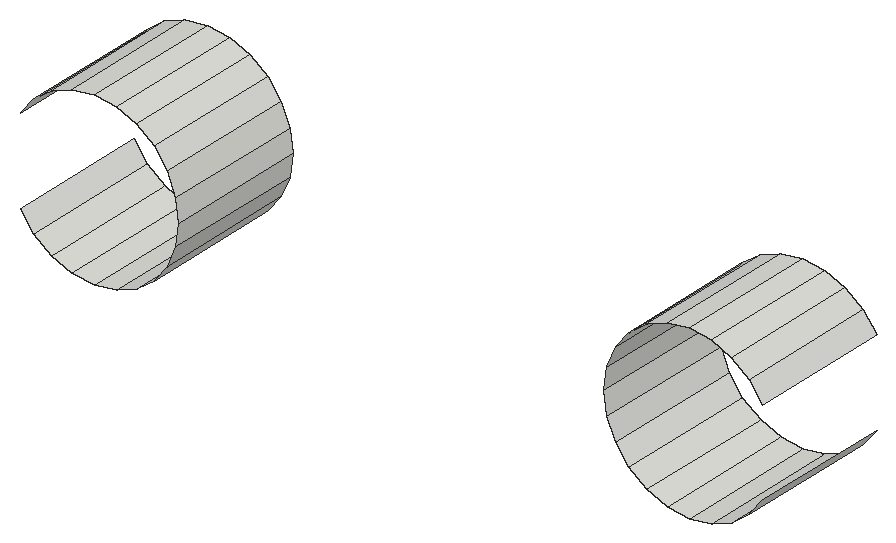
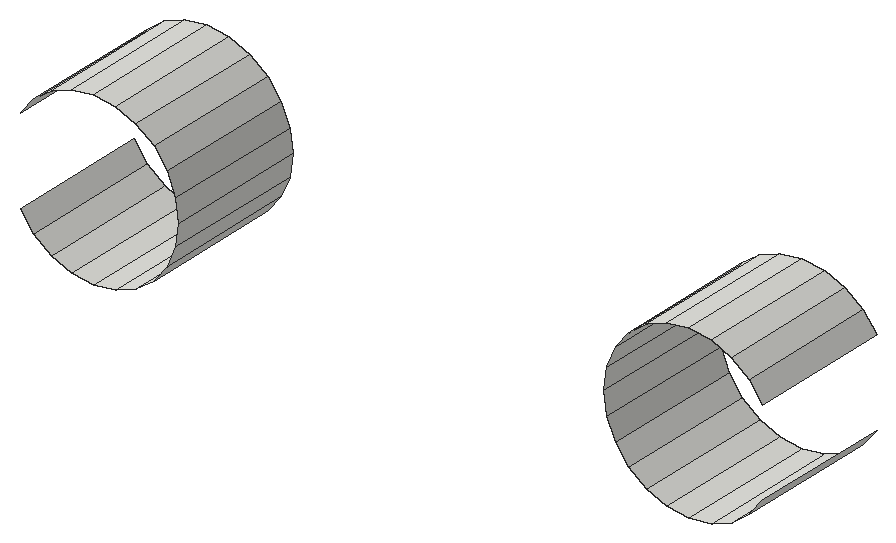
# SketchUp Ruby script. Lengths in inches.
U = 1.inch
M = Sketchup.active_model
def pt(a) = Geom::Point3d.new(a.map { |v| v * U })
def face(e, loops, mat)
  f = e.add_face(loops[0].map { |a| pt(a) })
  loops[1..].each { |l| e.add_face(l.map { |a| pt(a) }).erase! }
  f.material = f.back_material = mat if mat
  f
end
# faces: each face lists its corners as indices into pts; further lists are holes
def faces(e, pts, list, mat = nil) = list.each { |f| face(e, (f[0].is_a?(Array) ? f : [f]).map { |l| l.map { |i| pts[i] } }, mat) }
# xy, xz, yz: faces in a plane at the given z, y or x. An outline is a flat list of corners, or four numbers for a rectangle; further outlines are holes
def ring(l) = l.size == 4 ? [[l[0], l[1]], [l[2], l[1]], [l[2], l[3]], [l[0], l[3]]] : l.each_slice(2).to_a
def flat(e, list, mat, &to3) = list.each { |f| face(e, (f[0].is_a?(Array) ? f : [f]).map { |l| ring(l).map { |u, v| to3.(u, v) } }, mat) }
def xy(e, z, list, mat = nil) = flat(e, list, mat) { |x, y| [x, y, z] }
def xz(e, y, list, mat = nil) = flat(e, list, mat) { |x, z| [x, y, z] }
def yz(e, x, list, mat = nil) = flat(e, list, mat) { |y, z| [x, y, z] }
def lines(e, pts, list) = list.each { |a, b| e.add_line(pt(pts[a]), pt(pts[b])) }
# prism: a flat outline (further loops are holes) pulled along v
def prism(e, loops, v, mat = nil)
  f = face(e, loops, mat); d = Geom::Vector3d.new(v.map { |x| x * U })
  f.pushpull(f.normal.samedirection?(d) ? d.length : -d.length)
end
def box(e, o, s, mat = nil) = prism(e, [[o, [o[0] + s[0], o[1], o[2]], [o[0] + s[0], o[1] + s[1], o[2]], [o[0], o[1] + s[1], o[2]]]], [0, 0, s[2]], mat)
def at(x, y, z, deg = 0) = Geom::Transformation.translation(pt([x, y, z])) * Geom::Transformation.rotation(ORIGIN, Z_AXIS, deg.degrees)
def axes(o, x, y, z) = Geom::Transformation.new([*x, 0, *y, 0, *z, 0, *pt(o).to_a, 1])
def part(name) = M.definitions.add(name)
# library, detail: a bought-in or finely detailed component or shape, given as its bounding box
def library(name, o, s) = part(name).tap { |d| box(d.entities, o, s) }
def detail(e, o, s) = box(e.add_group.entities, o, s)
def put(e, d, t, mat = nil) = e.add_instance(d, t).tap { |i| i.material = mat if mat }
def group(e, t, mat = nil) = e.add_group.tap { |g| g.transformation = t; g.material = mat if mat }.entities
root = M.entities
p = [[3543,801.78,132.03],[3543.27,801.78,131.92],[3543.27,799.91,131.92],[3543,799.91,132.03],[3543.57,801.78,131.88],[3543.57,799.91,131.88],
  [3543.86,801.78,131.92],[3543.86,799.91,131.92],[3544.13,801.78,132.03],[3544.13,799.91,132.03],[3550.87,801.78,132.03],[3551.14,801.78,131.92],
  [3551.14,799.91,131.92],[3550.87,799.91,132.03],[3551.43,801.78,131.88],[3551.43,799.91,131.88],[3551.72,801.78,131.92],[3551.72,799.91,131.92],
  [3551.99,801.78,132.03],[3551.99,799.91,132.03],[3542.77,801.78,132.21],[3542.77,799.91,132.21],[3544.36,801.78,132.21],[3544.36,799.91,132.21],
  [3550.63,801.78,132.21],[3550.63,799.91,132.21],[3552.22,801.78,132.21],[3552.22,799.91,132.21],[3542.59,801.78,132.44],[3542.59,799.91,132.44],
  [3544.54,801.78,132.44],[3544.54,799.91,132.44],[3550.45,801.78,132.44],[3550.45,799.91,132.44],[3552.4,801.78,132.44],[3552.4,799.91,132.44],
  [3544.65,801.78,132.71],[3544.65,799.91,132.71],[3550.34,801.78,132.71],[3550.34,799.91,132.71],[3544.69,801.78,133],[3544.69,799.91,133],
  [3550.3,801.78,133],[3550.3,799.91,133],[3544.65,801.78,133.29],[3544.65,799.91,133.29],[3550.34,801.78,133.29],[3550.34,799.91,133.29],
  [3544.54,801.78,133.57],[3544.54,799.91,133.57],[3550.45,801.78,133.57],[3550.45,799.91,133.57],[3542.77,801.78,133.8],[3542.59,801.78,133.57],
  [3542.59,799.91,133.57],[3542.77,799.91,133.8],[3544.36,801.78,133.8],[3544.36,799.91,133.8],[3550.63,801.78,133.8],[3550.63,799.91,133.8],
  [3552.4,801.78,133.57],[3552.22,801.78,133.8],[3552.22,799.91,133.8],[3552.4,799.91,133.57],[3543,801.78,133.98],[3543,799.91,133.98],
  [3544.13,801.78,133.98],[3544.13,799.91,133.98],[3550.87,801.78,133.98],[3550.87,799.91,133.98],[3551.99,801.78,133.98],[3551.99,799.91,133.98],
  [3543.27,801.78,134.09],[3543.27,799.91,134.09],[3543.86,801.78,134.09],[3543.86,799.91,134.09],[3551.14,801.78,134.09],[3551.14,799.91,134.09],
  [3551.72,801.78,134.09],[3551.72,799.91,134.09],[3543.57,801.78,134.13],[3543.57,799.91,134.13],[3551.43,801.78,134.13],[3551.43,799.91,134.13]]
faces(root,p,[[0,1,2,3],[1,4,5,2],[4,6,7,5],[6,8,9,7],[10,11,12,13],[11,14,15,12],[14,16,17,15],[16,18,19,17],
  [20,0,3,21],[8,22,23,9],[24,10,13,25],[18,26,27,19],[28,20,21,29],[22,30,31,23],[32,24,25,33],[26,34,35,27],
  [30,36,37,31],[38,32,33,39],[36,40,41,37],[42,38,39,43],[40,44,45,41],[46,42,43,47],[44,48,49,45],[50,46,47,51],
  [52,53,54,55],[48,56,57,49],[58,50,51,59],[60,61,62,63],[64,52,55,65],[56,66,67,57],[68,58,59,69],[61,70,71,62],
  [72,64,65,73],[66,74,75,67],[76,68,69,77],[70,78,79,71],[80,72,73,81],[74,80,81,75],[82,76,77,83],[78,82,83,79]])
